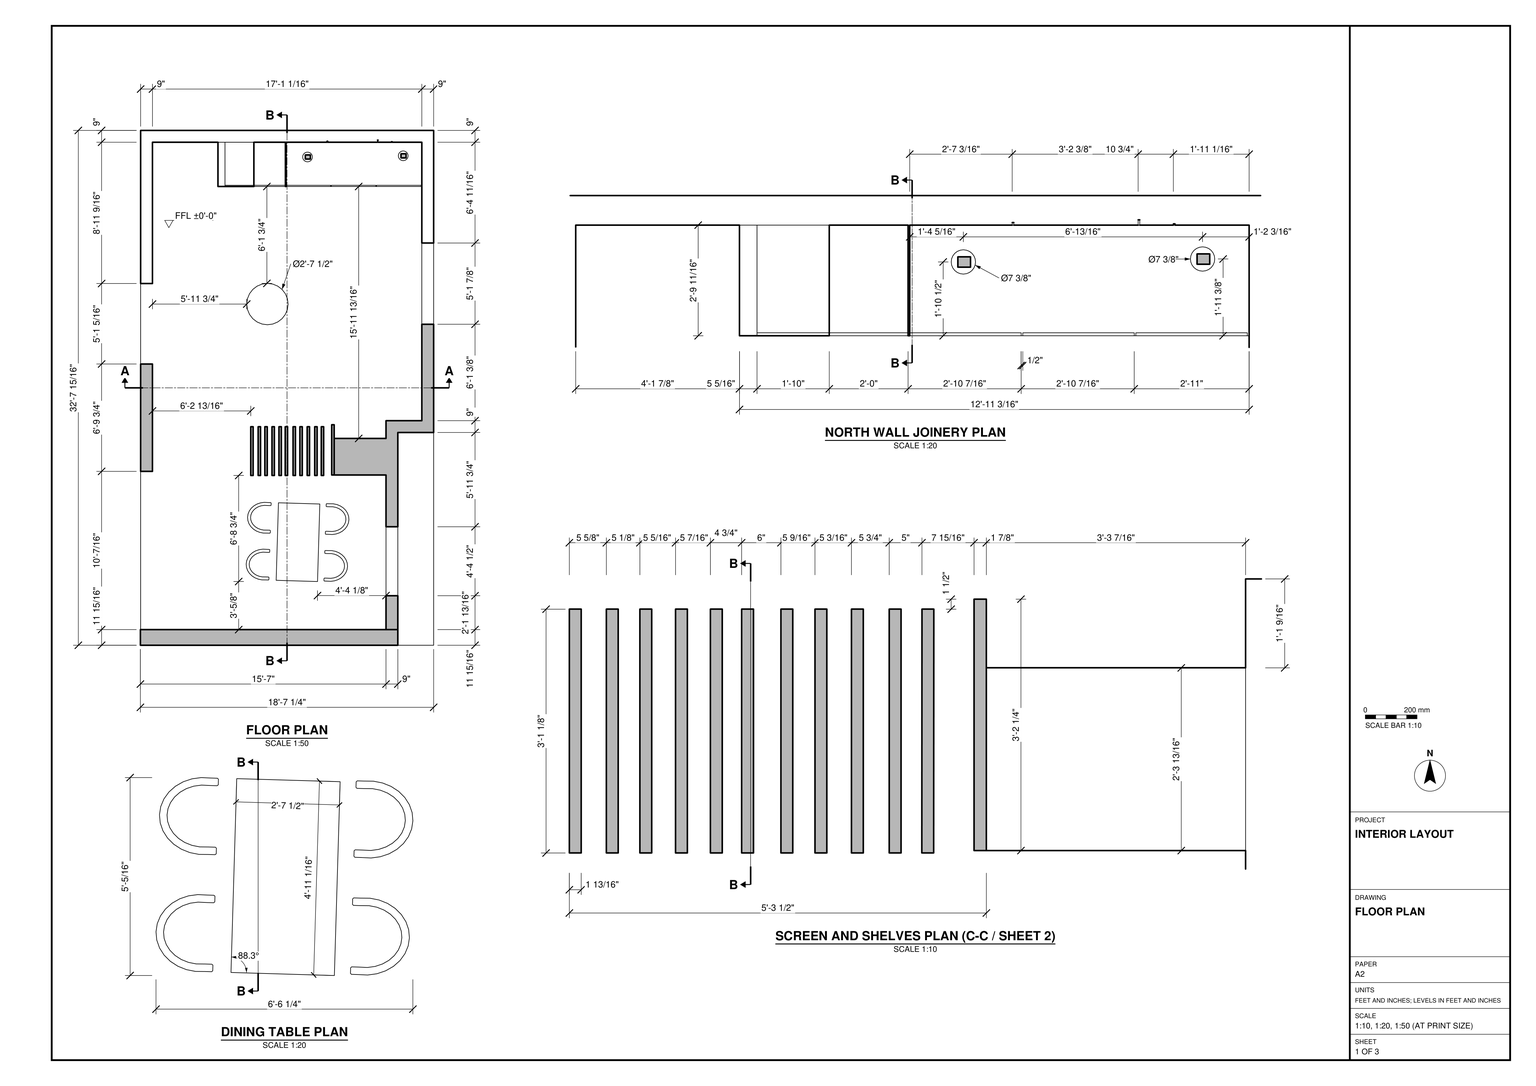
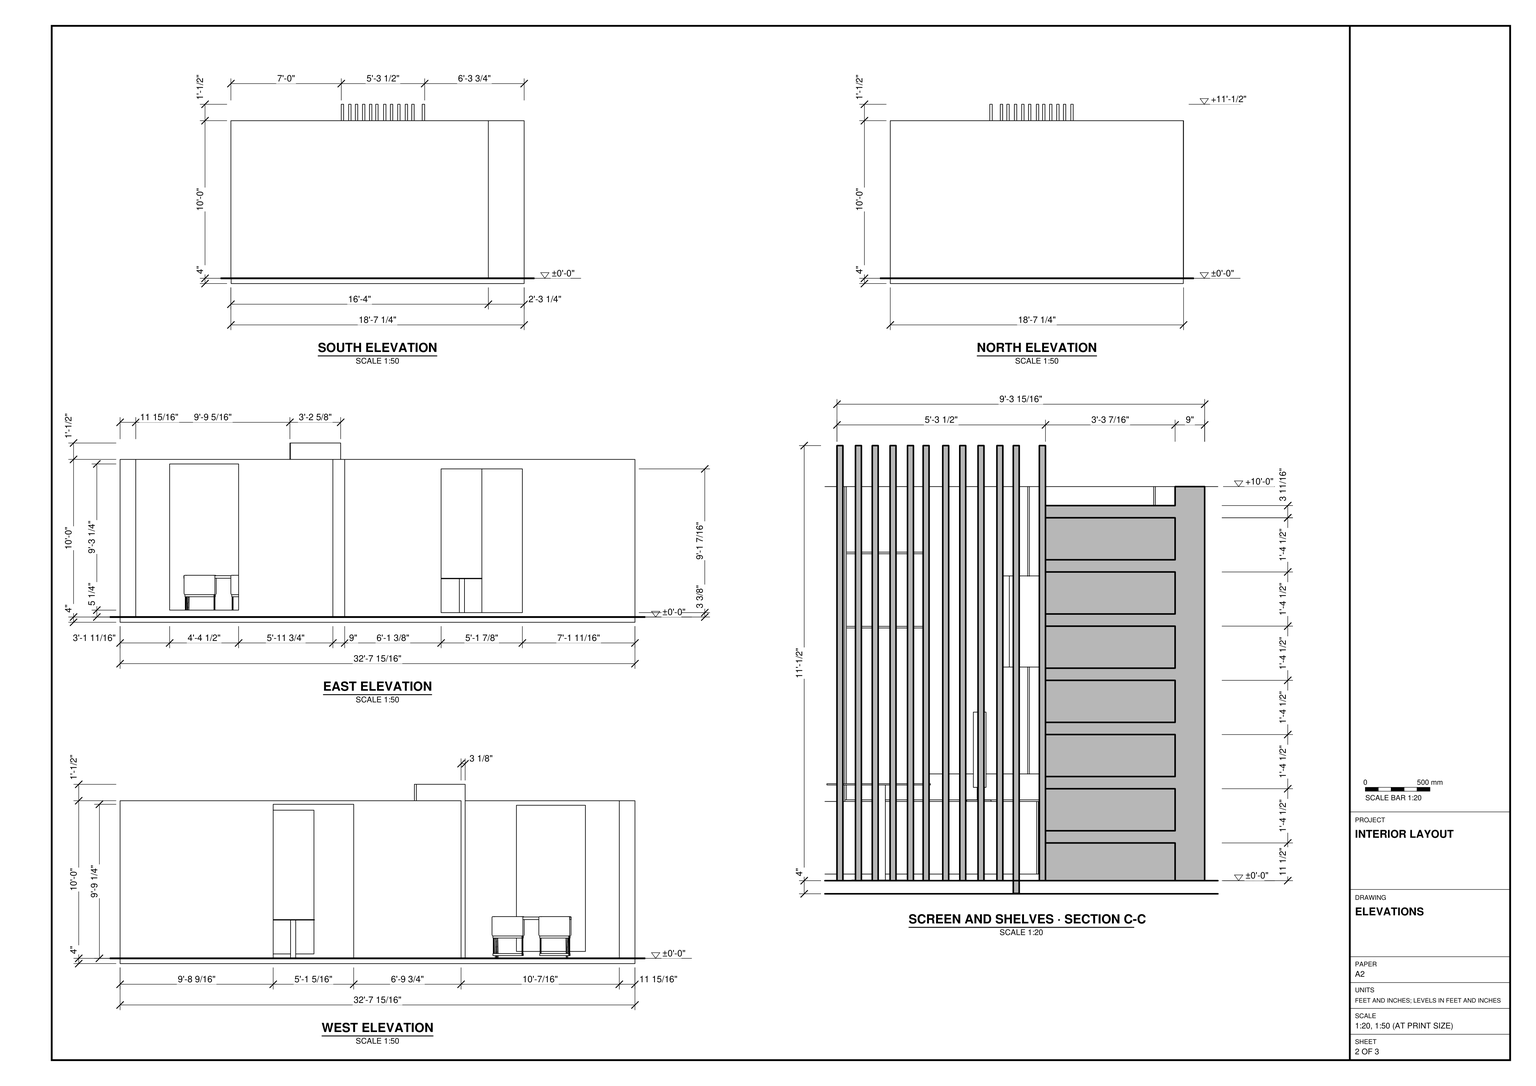
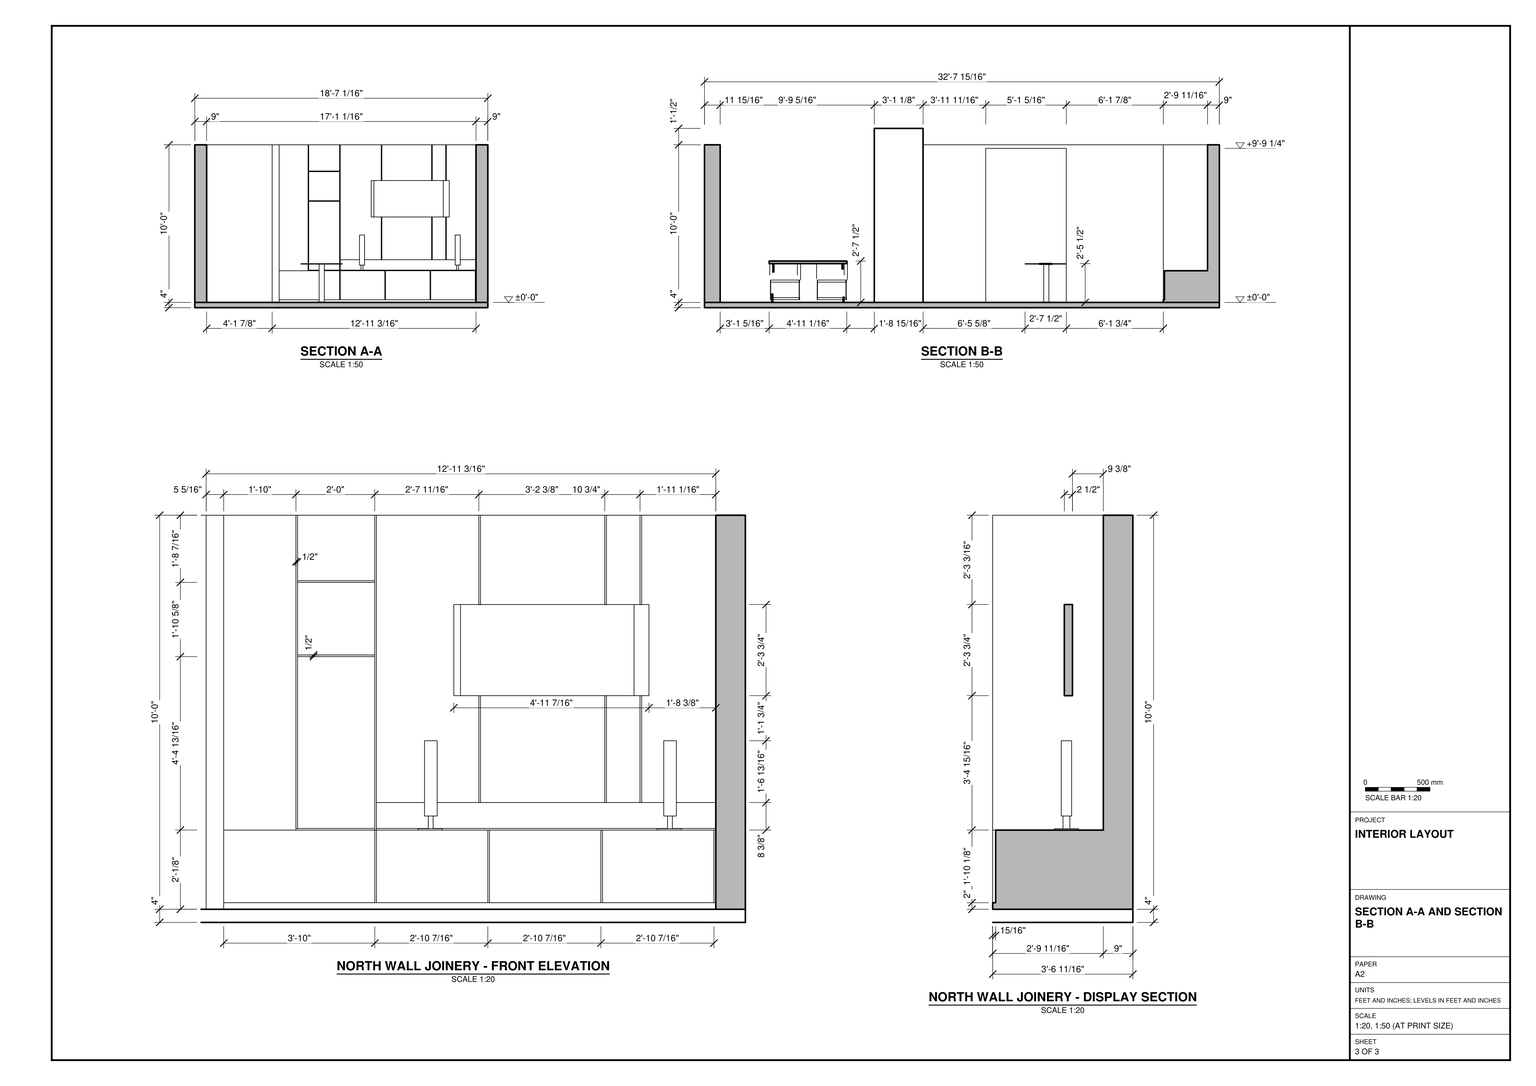
Use task_files/diagram_01.pdf to build the interior in SketchUp. Work in feet and inches. The overall model is 18'-7 1/4" east to west, 32'-7 15/16" north to south and 11'-4 1/2" high. Set the single finished floor level at ±0'-0", with the 4" floor slab below it. Follow the wall thicknesses in plan, including the 9" north wall and the stepped east wall beside the dining area. Use the east and west elevations to set the widths, sills and heads of the side openings.

Fit the display joinery against the north wall, leaving the west end of that wall clear. Model the divided base cabinets, narrow shelving bay, vertical backing panels and television in the arrangement shown in Section A-A and the joinery details. Place the round pedestal table between the display and the slatted screen. Run the screen across part of the room, with its fins projecting above the wall tops and stacked shelves connecting its east end to the wall. On the south side of the screen, place the rectangular dining table and four chairs at the slight angle shown in the dining table plan. Decor and loose items may be any suitable library components.

Keep the slab, walls and each furniture or joinery piece in separate groups or components, and use components for repeated parts. Save one SketchUp model as output_files/dining_and_display_interior_with_a_slatted_screen.skp.

# SketchUp Ruby script. Lengths in inches.
U = 1.inch
M = Sketchup.active_model
def pt(a) = Geom::Point3d.new(a.map { |v| v * U })
def face(e, loops, mat)
  f = e.add_face(loops[0].map { |a| pt(a) })
  loops[1..].each { |l| e.add_face(l.map { |a| pt(a) }).erase! }
  f.material = f.back_material = mat if mat
  f
end
# faces: each face lists its corners as indices into pts; further lists are holes
def faces(e, pts, list, mat = nil) = list.each { |f| face(e, (f[0].is_a?(Array) ? f : [f]).map { |l| l.map { |i| pts[i] } }, mat) }
# xy, xz, yz: faces in a plane at the given z, y or x. An outline is a flat list of corners, or four numbers for a rectangle; further outlines are holes
def ring(l) = l.size == 4 ? [[l[0], l[1]], [l[2], l[1]], [l[2], l[3]], [l[0], l[3]]] : l.each_slice(2).to_a
def flat(e, list, mat, &to3) = list.each { |f| face(e, (f[0].is_a?(Array) ? f : [f]).map { |l| ring(l).map { |u, v| to3.(u, v) } }, mat) }
def xy(e, z, list, mat = nil) = flat(e, list, mat) { |x, y| [x, y, z] }
def xz(e, y, list, mat = nil) = flat(e, list, mat) { |x, z| [x, y, z] }
def yz(e, x, list, mat = nil) = flat(e, list, mat) { |y, z| [x, y, z] }
def lines(e, pts, list) = list.each { |a, b| e.add_line(pt(pts[a]), pt(pts[b])) }
# prism: a flat outline (further loops are holes) pulled along v
def prism(e, loops, v, mat = nil)
  f = face(e, loops, mat); d = Geom::Vector3d.new(v.map { |x| x * U })
  f.pushpull(f.normal.samedirection?(d) ? d.length : -d.length)
end
def box(e, o, s, mat = nil) = prism(e, [[o, [o[0] + s[0], o[1], o[2]], [o[0] + s[0], o[1] + s[1], o[2]], [o[0], o[1] + s[1], o[2]]]], [0, 0, s[2]], mat)
def at(x, y, z, deg = 0) = Geom::Transformation.translation(pt([x, y, z])) * Geom::Transformation.rotation(ORIGIN, Z_AXIS, deg.degrees)
def axes(o, x, y, z) = Geom::Transformation.new([*x, 0, *y, 0, *z, 0, *pt(o).to_a, 1])
def part(name) = M.definitions.add(name)
# library, detail: a bought-in or finely detailed component or shape, given as its bounding box
def library(name, o, s) = part(name).tap { |d| box(d.entities, o, s) }
def detail(e, o, s) = box(e.add_group.entities, o, s)
def put(e, d, t, mat = nil) = e.add_instance(d, t).tap { |i| i.material = mat if mat }
def group(e, t, mat = nil) = e.add_group.tap { |g| g.transformation = t; g.material = mat if mat }.entities
root = M.entities
M.materials.add("Asphalt_06_1K").color = [164, 157, 139]
M.materials.add("Plywood_01_1K").color = [125, 96, 64]
M.materials.add("Wood_Planks_01_1K").color = [69, 67, 63]
M.materials.add("Wood_Veneer_15_1K").color = [103, 69, 45]
M.materials.add("[Color_007]").color = [58, 58, 58]
M.materials.add("[Color_008]").color = [30, 30, 30]
M.materials.add("[Color_009]").color = [0, 0, 0]
M.materials.add("[Color_A01]").color = [255, 0, 0]
c1 = library("Vienna Gold Table",[46.52,29.43,0],[31.5,31.5,29.53])
c2 = library("DinningTable",[0,0,0],[59.51,77.19,31.79])
c3 = part("Tv")
xy(c3.entities,0,[[2.03,0,1.74,0.06,1.46,0.15,1.19,0.27,0.95,0.43,0.72,0.62,0.52,0.84,0.35,1.08,0.21,1.34,0.1,1.61,0.03,1.9,0,2.19,0.01,2.48,59.41,2.48,59.17,2.1,58.9,1.74,58.59,1.41,58.25,1.1,57.89,0.83,57.5,0.6,57.09,0.4,56.67,0.24,56.23,0.12,55.78,0.04,55.33,0]],"[Color_009]")
xy(c3.entities,27.76,[[2.03,0,55.33,0,55.78,0.04,56.23,0.12,56.67,0.24,57.09,0.4,57.5,0.6,57.89,0.83,58.25,1.1,58.59,1.41,58.9,1.74,59.17,2.1,59.41,2.48,0.01,2.48,0,2.19,0.03,1.9,0.1,1.61,0.21,1.34,0.35,1.08,0.52,0.84,0.72,0.62,0.95,0.43,1.19,0.27,1.46,0.15,1.74,0.06]],"[Color_009]")
xz(c3.entities,0,[[2.03,0,54.875,27.76],[54.875,0,55.33,27.76]],"[Color_009]")
xz(c3.entities,2.48,[[0.69,0.6875,58.73,27.07]],"[Color_007]")
xz(c3.entities,2.48,[[[0.01,0,59.41,27.76],[0.69,0.6875,58.73,27.07],[5.81,0.12,5.86,0.12,5.91,0.13,5.99,0.19,6.03,0.29,6.03,0.34,6.01,0.39,5.99,0.43,5.95,0.47,5.91,0.5,5.86,0.51,5.81,0.51,5.76,0.5,5.71,0.47,5.65,0.39,5.64,0.34,5.64,0.29,5.65,0.24,5.68,0.19,5.71,0.16,5.76,0.13]]],"[Color_009]")
xz(c3.entities,2.48,[[5.81,0.12,5.76,0.13,5.71,0.16,5.68,0.19,5.65,0.24,5.64,0.29,5.64,0.34,5.65,0.39,5.71,0.47,5.76,0.5,5.81,0.51,5.86,0.51,5.91,0.5,5.95,0.47,5.99,0.43,6.01,0.39,6.03,0.34,6.03,0.29,5.99,0.19,5.91,0.13,5.86,0.12]],"[Color_A01]")
p = [[1.74,0.06,0],[2.03,0,0],[2.03,0,27.76],[1.74,0.06,27.76],[55.33,0,0],[55.78,0.04,0],
  [55.78,0.04,27.76],[55.33,0,27.76],[56.23,0.12,0],[56.23,0.12,27.76],[1.19,0.27,0],[1.46,0.15,0],
  [1.46,0.15,27.76],[1.19,0.27,27.76],[56.67,0.24,0],[56.67,0.24,27.76],[57.09,0.4,0],[57.09,0.4,27.76],
  [0.95,0.43,0],[0.95,0.43,27.76],[0.72,0.62,0],[0.72,0.62,27.76],[57.5,0.6,0],[57.5,0.6,27.76],
  [0.52,0.84,0],[0.52,0.84,27.76],[57.89,0.83,0],[57.89,0.83,27.76],[0.35,1.08,0],[0.35,1.08,27.76],
  [58.25,1.1,0],[58.25,1.1,27.76],[0.21,1.34,0],[0.21,1.34,27.76],[58.59,1.41,0],[58.59,1.41,27.76],
  [0.1,1.61,0],[0.1,1.61,27.76],[58.9,1.74,0],[58.9,1.74,27.76],[0.03,1.9,0],[0.03,1.9,27.76],
  [59.17,2.1,0],[59.17,2.1,27.76],[0,2.19,0],[0,2.19,27.76],[59.41,2.48,0],[59.41,2.48,27.76],
  [0.01,2.48,0],[0.01,2.48,27.76]]
faces(c3.entities,p,[[0,1,2,3],[4,5,6,7],[5,8,9,6],[10,11,12,13],[11,0,3,12],[8,14,15,9],[14,16,17,15],[18,10,13,19],
  [20,18,19,21],[16,22,23,17],[24,20,21,25],[22,26,27,23],[28,24,25,29],[26,30,31,27],[32,28,29,33],[30,34,35,31],
  [36,32,33,37],[34,38,39,35],[40,36,37,41],[38,42,43,39],[44,40,41,45],[42,46,47,43],[48,44,45,49]],"[Color_009]")
c4 = part("Televisão")
xy(c4.entities,0,[[3.7,0,2.74,0.125,1.85,0.5,1.08,1.08,0.5,1.85,0.125,2.74,0,3.7,0.125,4.66,0.5,5.55,1.08,6.32,1.85,6.91,2.74,7.28,3.7,7.4,4.66,7.28,5.55,6.91,6.32,6.32,6.91,5.55,7.28,4.66,7.4,3.7,7.28,2.74,6.91,1.85,6.32,1.08,5.55,0.5,4.66,0.125],[76.54,0.89,75.59,1.02,74.69,1.39,73.93,1.98,73.34,2.74,72.97,3.64,72.84,4.59,72.97,5.55,73.34,6.44,73.93,7.21,74.69,7.8,75.59,8.17,76.54,8.29,77.5,8.17,78.39,7.8,79.16,7.21,79.75,6.44,80.12,5.55,80.24,4.59,80.12,3.64,79.75,2.74,79.16,1.98,78.39,1.39,77.5,1.02]],"[Color_009]")
xy(c4.entities,0.43,[[[3.7,0,4.66,0.125,5.55,0.5,6.32,1.08,6.91,1.85,7.28,2.74,7.4,3.7,7.28,4.66,6.91,5.55,6.32,6.32,5.55,6.91,4.66,7.28,3.7,7.4,2.74,7.28,1.85,6.91,1.08,6.32,0.5,5.55,0.125,4.66,0,3.7,0.125,2.74,0.5,1.85,1.08,1.08,1.85,0.5,2.74,0.125],[3.18,2.63,4.64,4.72]],[[76.54,0.89,77.5,1.02,78.39,1.39,79.16,1.98,79.75,2.74,80.12,3.64,80.24,4.59,80.12,5.55,79.75,6.44,79.16,7.21,78.39,7.8,77.5,8.17,76.54,8.29,75.59,8.17,74.69,7.8,73.93,7.21,73.34,6.44,72.97,5.55,72.84,4.59,72.97,3.64,73.34,2.74,73.93,1.98,74.69,1.39,75.59,1.02],[76.03,3.53,77.48,5.61]]],"[Color_008]")
xy(c4.entities,4.29,[[[2.02,2.1,5.88,5.25],[3.18,2.63,4.64,4.72]],[[74.87,2.99,78.72,6.14],[76.03,3.53,77.48,5.61]]],"[Color_009]")
xy(c4.entities,27.2,[[2.02,2.1,5.88,5.25],[74.87,2.99,78.72,6.14]],"[Color_009]")
xz(c4.entities,2.1,[[2.02,4.29,5.88,27.2]],"[Color_009]")
xz(c4.entities,2.63,[[3.18,0.43,4.64,4.29]],"[Color_009]")
xz(c4.entities,2.99,[[74.87,4.29,78.72,27.2]],"[Color_009]")
xz(c4.entities,3.53,[[76.03,0.43,77.48,4.29]],"[Color_009]")
xz(c4.entities,4.72,[[3.18,0.43,4.64,4.29]],"[Color_009]")
xz(c4.entities,5.25,[[2.17,4.44,5.73,27.06]],"[Color_007]")
xz(c4.entities,5.25,[[[2.02,4.29,5.88,27.2],[2.17,4.44,5.73,27.06]]],"[Color_009]")
xz(c4.entities,5.61,[[76.03,0.43,77.48,4.29]],"[Color_009]")
xz(c4.entities,6.14,[[75.01,4.44,78.58,27.06]],"[Color_007]")
xz(c4.entities,6.14,[[[74.87,4.29,78.72,27.2],[75.01,4.44,78.58,27.06]]],"[Color_009]")
yz(c4.entities,2.02,[[2.1,4.29,5.25,27.2]],"[Color_009]")
yz(c4.entities,3.18,[[2.63,0.43,4.72,4.29]],"[Color_009]")
yz(c4.entities,4.64,[[2.63,0.43,4.72,4.29]],"[Color_009]")
yz(c4.entities,5.88,[[2.1,4.29,5.25,27.2]],"[Color_009]")
yz(c4.entities,74.87,[[2.99,4.29,6.14,27.2]],"[Color_009]")
yz(c4.entities,76.03,[[3.53,0.43,5.61,4.29]],"[Color_009]")
yz(c4.entities,77.48,[[3.53,0.43,5.61,4.29]],"[Color_009]")
yz(c4.entities,78.72,[[2.99,4.29,6.14,27.2]],"[Color_009]")
p = [[2.74,0.125,0],[3.7,0,0],[3.7,0,0.43],[2.74,0.125,0.43],[4.66,0.125,0],[4.66,0.125,0.43],
  [1.85,0.5,0],[1.85,0.5,0.43],[5.55,0.5,0],[5.55,0.5,0.43],[1.08,1.08,0],[1.08,1.08,0.43],
  [6.32,1.08,0],[6.32,1.08,0.43],[75.59,1.02,0],[76.54,0.89,0],[76.54,0.89,0.43],[75.59,1.02,0.43],
  [77.5,1.02,0],[77.5,1.02,0.43],[74.69,1.39,0],[74.69,1.39,0.43],[78.39,1.39,0],[78.39,1.39,0.43],
  [0.5,1.85,0],[0.5,1.85,0.43],[6.91,1.85,0],[6.91,1.85,0.43],[73.93,1.98,0],[73.93,1.98,0.43],
  [79.16,1.98,0],[79.16,1.98,0.43],[0.125,2.74,0],[0.125,2.74,0.43],[7.28,2.74,0],[7.28,2.74,0.43],
  [73.34,2.74,0],[73.34,2.74,0.43],[79.75,2.74,0],[79.75,2.74,0.43],[0,3.7,0],[0,3.7,0.43],
  [7.4,3.7,0],[7.4,3.7,0.43],[72.97,3.64,0],[72.97,3.64,0.43],[80.12,3.64,0],[80.12,3.64,0.43],
  [72.84,4.59,0],[72.84,4.59,0.43],[80.24,4.59,0],[80.24,4.59,0.43],[0.125,4.66,0],[0.125,4.66,0.43],
  [7.28,4.66,0],[7.28,4.66,0.43],[72.97,5.55,0],[72.97,5.55,0.43],[80.12,5.55,0],[80.12,5.55,0.43],
  [0.5,5.55,0],[0.5,5.55,0.43],[6.91,5.55,0],[6.91,5.55,0.43],[1.08,6.32,0],[1.08,6.32,0.43],
  [6.32,6.32,0],[6.32,6.32,0.43],[73.34,6.44,0],[73.34,6.44,0.43],[79.75,6.44,0],[79.75,6.44,0.43],
  [1.85,6.91,0],[1.85,6.91,0.43],[5.55,6.91,0],[5.55,6.91,0.43],[73.93,7.21,0],[73.93,7.21,0.43],
  [79.16,7.21,0],[79.16,7.21,0.43],[2.74,7.28,0],[2.74,7.28,0.43],[4.66,7.28,0],[4.66,7.28,0.43],
  [74.69,7.8,0],[74.69,7.8,0.43],[78.39,7.8,0],[78.39,7.8,0.43],[3.7,7.4,0],[3.7,7.4,0.43],
  [75.59,8.17,0],[75.59,8.17,0.43],[77.5,8.17,0],[77.5,8.17,0.43],[76.54,8.29,0],[76.54,8.29,0.43],
  [75.4,3.53,4.29],[75.4,3.53,20.55],[77.48,5.61,4.29],[77.48,5.61,20.55],[75.4,5.61,4.29],[75.4,5.61,20.55],
  [2.55,2.63,4.29],[2.55,2.63,20.55],[4.64,4.72,4.29],[4.64,4.72,20.55],[2.55,4.72,4.29],[2.55,4.72,20.55]]
faces(c4.entities,p,[[0,1,2,3],[1,4,5,2],[6,0,3,7],[4,8,9,5],[10,6,7,11],[8,12,13,9],[14,15,16,17],[15,18,19,16],
  [20,14,17,21],[18,22,23,19],[24,10,11,25],[12,26,27,13],[28,20,21,29],[22,30,31,23],[32,24,25,33],[26,34,35,27],
  [36,28,29,37],[30,38,39,31],[40,32,33,41],[34,42,43,35],[44,36,37,45],[38,46,47,39],[48,44,45,49],[46,50,51,47],
  [52,40,41,53],[42,54,55,43],[56,48,49,57],[50,58,59,51],[60,52,53,61],[54,62,63,55],[64,60,61,65],[62,66,67,63],
  [68,56,57,69],[58,70,71,59],[72,64,65,73],[66,74,75,67],[76,68,69,77],[70,78,79,71],[80,72,73,81],[74,82,83,75],
  [84,76,77,85],[78,86,87,79],[88,80,81,89],[82,88,89,83],[90,84,85,91],[86,92,93,87],[94,90,91,95],[92,94,95,93]],"[Color_009]")
lines(c4.entities,p,[[96,97],[98,99],[100,101],[102,103],[104,105],[106,107]])
put(c4.entities,c3,at(10.94,3.03,40.93))
xy(root,0.12,[[137.68,129.27,137.71,166.4,139.51,166.4,139.49,129.27]])
xy(root,4,[[0,0,186.98,11.93],[186.98,11.93,186.98,170.99,214.24,170.99,214.24,382.95,9.19,382.95,9.19,275.4,0.19,275.4,0.19,391.95,223.24,391.95,223.24,161.99,195.98,161.99,195.98,11.93],[84.02,129.27,85.82,166.4],[89.65,129.27,91.46,166.4],[94.76,129.27,96.5625,166.4],
  [100.1875,129.27,101.99,166.4],[105.49,129.27,107.3,166.4],[110.25,129.27,112.06,166.4],[116.23,129.27,118.04,166.4],[121.42,129.27,123.22,166.4],
  [126.97,129.27,128.77,166.4],[132.72,129.27,134.52,166.4],[145.64,129.63,147.51,167.91],[0.19,132.38,9.19,214.11],[59.05,349.26,64.39,382.95],
  [64.39,349.26,214.24,382.95]])
xy(root,6,[[64.39,349.26,110.41,350.17],[110.91,349.26,144.83,350.17],[145.33,349.26,179.25,350.17],[179.75,349.26,213.67,350.17]],"Plywood_01_1K")
xy(root,7.36,[[214.24,244.38,223.24,306.23]])
xy(root,9.26,[[186.98,37.72,195.98,90.23]])
xy(root,15.49,[[147.51,129.63,186.98,157.46]],"Wood_Veneer_15_1K")
xy(root,19.19,[[147.51,129.63,186.98,157.46]],"Wood_Veneer_15_1K")
xy(root,28.11,[[64.39,349.26,86.39,350.17],[110.39,349.26,110.41,350.17],[110.41,349.26,110.41,350.17,110.39,350.17,110.39,382.95,110.89,382.95,110.89,349.26]])
xy(root,28.11,[[110.89,349.26,110.91,349.26,110.91,350.17,144.83,350.17,144.83,349.26,145.33,349.26,145.33,350.17,179.25,350.17,179.25,349.26,179.75,349.26,179.75,350.17,213.67,350.17,213.67,349.26,214.24,349.26,214.24,382.95,110.89,382.95],[86.39,350.17,110.39,382.95]],"Plywood_01_1K")
xy(root,28.61,[[142.09,382.95,142.59,383.73],[180.45,382.95,180.95,384.57],[191.17,382.95,191.67,383.34]])
xy(root,31.99,[[147.51,129.63,186.98,157.46]],"Wood_Veneer_15_1K")
xy(root,35.7,[[147.51,129.63,186.98,157.46]],"Wood_Veneer_15_1K")
xy(root,48.49,[[147.51,129.63,186.98,157.46]],"Wood_Veneer_15_1K")
xy(root,52.2,[[147.51,129.63,186.98,157.46]],"Wood_Veneer_15_1K")
xy(root,65,[[147.51,129.63,186.98,157.46]],"Wood_Veneer_15_1K")
xy(root,68.71,[[147.51,129.63,186.98,157.46]],"Wood_Veneer_15_1K")
xy(root,80.94,[[86.89,349.26,110.39,382.95]])
xy(root,81.44,[[86.89,349.26,110.39,382.95]],"Plywood_01_1K")
xy(root,81.5,[[147.51,129.63,186.98,157.46]],"Wood_Veneer_15_1K")
xy(root,85.21,[[147.51,129.63,186.98,157.46]],"Wood_Veneer_15_1K")
xy(root,98,[[147.51,129.63,186.98,157.46]],"Wood_Veneer_15_1K")
xy(root,101.71,[[147.51,129.63,186.98,157.46]],"Wood_Veneer_15_1K")
xy(root,103.54,[[86.89,349.26,110.39,382.95]],"Plywood_01_1K")
xy(root,104.04,[[86.89,349.26,110.39,382.95]],"Plywood_01_1K")
xy(root,114.51,[[147.51,129.63,186.98,157.46]],"Wood_Veneer_15_1K")
xy(root,116.79,[[214.24,244.38,223.24,306.23]])
xy(root,118.22,[[147.51,129.63,186.98,157.46]],"Wood_Veneer_15_1K")
xy(root,120.53,[[186.98,37.72,195.98,90.23]])
xy(root,121.27,[[0.19,214.11,9.19,275.4]])
xy(root,124,[[186.98,11.93,195.98,11.93,195.98,161.99,223.24,161.99,223.24,170.99,186.98,170.99],[0.19,132.38,9.19,132.38,9.19,382.95,110.39,382.95,110.39,349.26,110.89,349.26,110.89,382.95,142.09,382.95,142.09,383.73,142.59,383.73,142.59,382.95,180.45,382.95,180.45,384.57,180.95,384.57,180.95,382.95,191.17,382.95,191.17,383.34,191.67,383.34,191.67,382.95,214.24,382.95,214.24,170.99,223.24,170.99,223.24,391.95,0.19,391.95],[59.05,349.26,64.39,382.95]])
xy(root,124,[[0,0,195.98,11.93],[64.39,349.26,86.39,382.95]],"Plywood_01_1K")
xy(root,136.49,[[84.02,129.27,85.82,166.4],[89.65,129.27,91.46,166.4],[94.76,129.27,96.5625,166.4],[100.1875,129.27,101.99,166.4],[105.49,129.27,107.3,166.4],
  [110.25,129.27,112.06,166.4],[116.23,129.27,118.04,166.4],[121.42,129.27,123.22,166.4],[126.97,129.27,128.77,166.4],[132.72,129.27,134.52,166.4],
  [137.68,129.27,139.49,129.27,139.51,166.4,137.71,166.4],[145.64,129.63,147.51,167.91]],"Wood_Planks_01_1K")
xz(root,0,[[0,4,195.98,124]])
xz(root,11.93,[[0,4,186.98,124],[186.98,4,195.98,124]])
xz(root,37.72,[[186.98,9.26,195.98,120.53]])
xz(root,90.23,[[186.98,9.26,195.98,120.53]])
xz(root,129.27,[[137.68,0.12,139.49,136.49],[84.02,4,85.82,136.49],[89.65,4,91.46,136.49],[94.76,4,96.5625,136.49],[100.1875,4,101.99,136.49],
  [105.49,4,107.3,136.49],[110.25,4,112.06,136.49],[116.23,4,118.04,136.49],[121.42,4,123.22,136.49],[126.97,4,128.77,136.49],
  [132.72,4,134.52,136.49]],"Wood_Planks_01_1K")
xz(root,129.63,[[145.64,4,147.51,136.49]],"Wood_Planks_01_1K")
xz(root,129.63,[[147.51,15.49,186.98,19.19],[147.51,31.99,186.98,35.7],[147.51,48.49,186.98,52.2],[147.51,65,186.98,68.71],[147.51,81.5,186.98,85.21],
  [147.51,98,186.98,101.71],[147.51,114.51,186.98,118.22]],"Wood_Veneer_15_1K")
xz(root,132.38,[[0.19,4,9.19,124]])
xz(root,157.46,[[147.51,15.49,186.98,19.19],[147.51,31.99,186.98,35.7],[147.51,48.49,186.98,52.2],[147.51,65,186.98,68.71],[147.51,81.5,186.98,85.21],
  [147.51,98,186.98,101.71],[147.51,114.51,186.98,118.22]])
xz(root,161.99,[[195.98,4,223.24,124]])
xz(root,166.4,[[137.71,0.12,139.51,136.49],[84.02,4,85.82,136.49],[89.65,4,91.46,136.49],[94.76,4,96.5625,136.49],[100.1875,4,101.99,136.49],
  [105.49,4,107.3,136.49],[110.25,4,112.06,136.49],[116.23,4,118.04,136.49],[121.42,4,123.22,136.49],[126.97,4,128.77,136.49],
  [132.72,4,134.52,136.49]])
xz(root,167.91,[[145.64,4,147.51,136.49]])
xz(root,170.99,[[186.98,4,214.24,124]])
xz(root,214.11,[[0.19,4,9.19,121.27]])
xz(root,244.38,[[214.24,7.36,223.24,116.79]])
xz(root,275.4,[[0.19,4,9.19,121.27]])
xz(root,306.23,[[214.24,7.36,223.24,116.79]])
xz(root,349.26,[[59.05,4,64.39,124]])
xz(root,349.26,[[64.39,4,214.24,6],[110.41,6,110.91,28.11],[144.83,6,145.33,28.11],[179.25,6,179.75,28.11],[213.67,6,214.24,28.11],
  [64.39,28.11,86.39,124],[110.39,28.11,110.89,124],[86.89,80.94,110.39,81.44],[86.89,103.54,110.39,104.04]],"Plywood_01_1K")
xz(root,350.17,[[64.39,6,110.41,28.11],[110.91,6,144.83,28.11],[145.33,6,179.25,28.11],[179.75,6,213.67,28.11]],"Plywood_01_1K")
xz(root,382.95,[[9.19,4,59.05,124]])
xz(root,382.95,[[110.89,36.51,142.09,124],[142.59,36.51,180.45,124],[180.95,36.51,191.17,124],[191.67,36.51,214.24,124]],"Asphalt_06_1K")
xz(root,382.95,[[86.39,28.11,110.39,28.61],[110.89,28.11,214.24,28.61],[86.39,28.61,86.89,124],[86.89,28.61,110.39,80.94],[110.89,28.61,214.24,36.51],
  [86.89,81.44,110.39,103.54],[86.89,104.04,110.39,124]],"Plywood_01_1K")
xz(root,383.34,[[191.17,28.61,191.67,124]])
xz(root,383.73,[[142.09,28.61,142.59,124]])
xz(root,384.57,[[180.45,28.61,180.95,124]])
xz(root,391.95,[[0.19,4,223.24,124]])
yz(root,0,[[0,4,11.93,124]])
yz(root,0.19,[[132.38,4,132.38,124,391.95,124,391.95,4,275.4,4,275.4,121.27,214.11,121.27,214.11,4]])
yz(root,9.19,[[132.38,4,141.38,124],[141.38,4,214.11,4,214.11,121.27,275.4,121.27,275.4,4,382.95,4,382.95,124,141.38,124]])
yz(root,59.05,[[349.26,4,382.95,124]])
yz(root,64.39,[[349.26,6,350.17,28.11]])
yz(root,84.02,[[129.27,4,166.4,136.49]],"Wood_Planks_01_1K")
yz(root,85.82,[[129.27,4,166.4,136.49]],"Wood_Planks_01_1K")
yz(root,86.39,[[349.26,28.11,382.95,124]],"Plywood_01_1K")
yz(root,86.89,[[349.26,80.94,382.95,81.44],[349.26,103.54,382.95,104.04]])
yz(root,89.65,[[129.27,4,166.4,136.49]],"Wood_Planks_01_1K")
yz(root,91.46,[[129.27,4,166.4,136.49]],"Wood_Planks_01_1K")
yz(root,94.76,[[129.27,4,166.4,136.49]],"Wood_Planks_01_1K")
yz(root,96.5625,[[129.27,4,166.4,136.49]],"Wood_Planks_01_1K")
yz(root,100.1875,[[129.27,4,166.4,136.49]],"Wood_Planks_01_1K")
yz(root,101.99,[[129.27,4,166.4,136.49]],"Wood_Planks_01_1K")
yz(root,105.49,[[129.27,4,166.4,136.49]],"Wood_Planks_01_1K")
yz(root,107.3,[[129.27,4,166.4,136.49]],"Wood_Planks_01_1K")
yz(root,110.25,[[129.27,4,166.4,136.49]],"Wood_Planks_01_1K")
yz(root,110.39,[[349.26,28.11,382.95,80.94],[349.26,81.44,382.95,103.54],[349.26,104.04,382.95,124]],"Plywood_01_1K")
yz(root,110.41,[[349.26,6,350.17,28.11]],"Plywood_01_1K")
yz(root,110.89,[[349.26,28.11,382.95,124]],"Plywood_01_1K")
yz(root,110.91,[[349.26,6,350.17,28.11]],"Plywood_01_1K")
yz(root,112.06,[[129.27,4,166.4,136.49]],"Wood_Planks_01_1K")
yz(root,116.23,[[129.27,4,166.4,136.49]],"Wood_Planks_01_1K")
yz(root,118.04,[[129.27,4,166.4,136.49]],"Wood_Planks_01_1K")
yz(root,121.42,[[129.27,4,166.4,136.49]],"Wood_Planks_01_1K")
yz(root,123.22,[[129.27,4,166.4,136.49]],"Wood_Planks_01_1K")
yz(root,126.97,[[129.27,4,166.4,136.49]],"Wood_Planks_01_1K")
yz(root,128.77,[[129.27,4,166.4,136.49]],"Wood_Planks_01_1K")
yz(root,132.72,[[129.27,4,166.4,136.49]],"Wood_Planks_01_1K")
yz(root,134.52,[[129.27,4,166.4,136.49]],"Wood_Planks_01_1K")
yz(root,144.83,[[349.26,6,350.17,28.11]])
yz(root,145.33,[[349.26,6,350.17,28.11]],"Plywood_01_1K")
yz(root,145.64,[[129.63,4,167.91,136.49]],"Wood_Planks_01_1K")
yz(root,147.51,[[129.63,15.49,157.46,19.19],[129.63,31.99,157.46,35.7],[129.63,48.49,157.46,52.2],[129.63,65,157.46,68.71],[129.63,81.5,157.46,85.21],
  [129.63,98,157.46,101.71],[129.63,114.51,157.46,118.22]])
yz(root,147.51,[[129.63,4,167.91,4,167.91,136.49,129.63,136.49,129.63,118.22,157.46,118.22,157.46,114.51,129.63,114.51,129.63,101.71,157.46,101.71,157.46,98,129.63,98,129.63,85.21,157.46,85.21,157.46,81.5,129.63,81.5,129.63,68.71,157.46,68.71,157.46,65,129.63,65,129.63,52.2,157.46,52.2,157.46,48.49,129.63,48.49,129.63,35.7,157.46,35.7,157.46,31.99,129.63,31.99,129.63,19.19,157.46,19.19,157.46,15.49,129.63,15.49]],"Wood_Planks_01_1K")
yz(root,179.25,[[349.26,6,350.17,28.11]])
yz(root,179.75,[[349.26,6,350.17,28.11]],"Plywood_01_1K")
yz(root,186.98,[[[11.93,4,170.99,124],[37.72,9.26,90.23,120.53],[129.63,114.51,157.46,118.22],[129.63,98,157.46,101.71],[129.63,81.5,157.46,85.21],[129.63,65,157.46,68.71],[129.63,48.49,157.46,52.2],[129.63,31.99,157.46,35.7],[129.63,15.49,157.46,19.19]]])
yz(root,195.98,[[0,4,11.93,124],[[11.93,4,161.99,124],[37.72,9.26,90.23,120.53]]])
yz(root,213.67,[[349.26,6,350.17,28.11]],"Plywood_01_1K")
yz(root,214.24,[[[170.99,4,170.99,124,382.95,124,382.95,28.11,349.26,28.11,349.26,4],[244.38,7.36,306.23,116.79]]])
yz(root,223.24,[[161.99,4,170.99,124],[[170.99,4,391.95,124],[244.38,7.36,306.23,116.79]]])
p = [[137.68,129.27,136.49],[137.71,166.4,136.49],[137.71,166.4,0.12],[137.68,129.27,0.12],[139.51,166.4,136.49],[139.49,129.27,136.49],
  [139.49,129.27,0.12],[139.51,166.4,0.12],[223.24,132.38,4],[223.24,161.99,4]]
faces(root,p,[[0,1,2,3],[4,5,6,7]],"Wood_Planks_01_1K")
lines(root,p,[[8,9]])
put(root,c1,at(34.43,214.59,4))
put(root,c2,at(157.33,47.86,4,88.3))
put(root,c4,at(123.52,368.04,28.11))
g1 = group(root,at(0.19,132.38,0))
xy(g1,0,[[0,-132.38,223.06,259.57]])
xy(g1,4,[[0,-132.38,223.06,259.57]],"Plywood_01_1K")
xz(g1,-132.38,[[0,0,223.06,4]])
xz(g1,259.57,[[0,0,223.06,4]])
yz(g1,0,[[-132.38,0,259.57,4]])
yz(g1,223.06,[[-132.38,0,259.57,4]])
